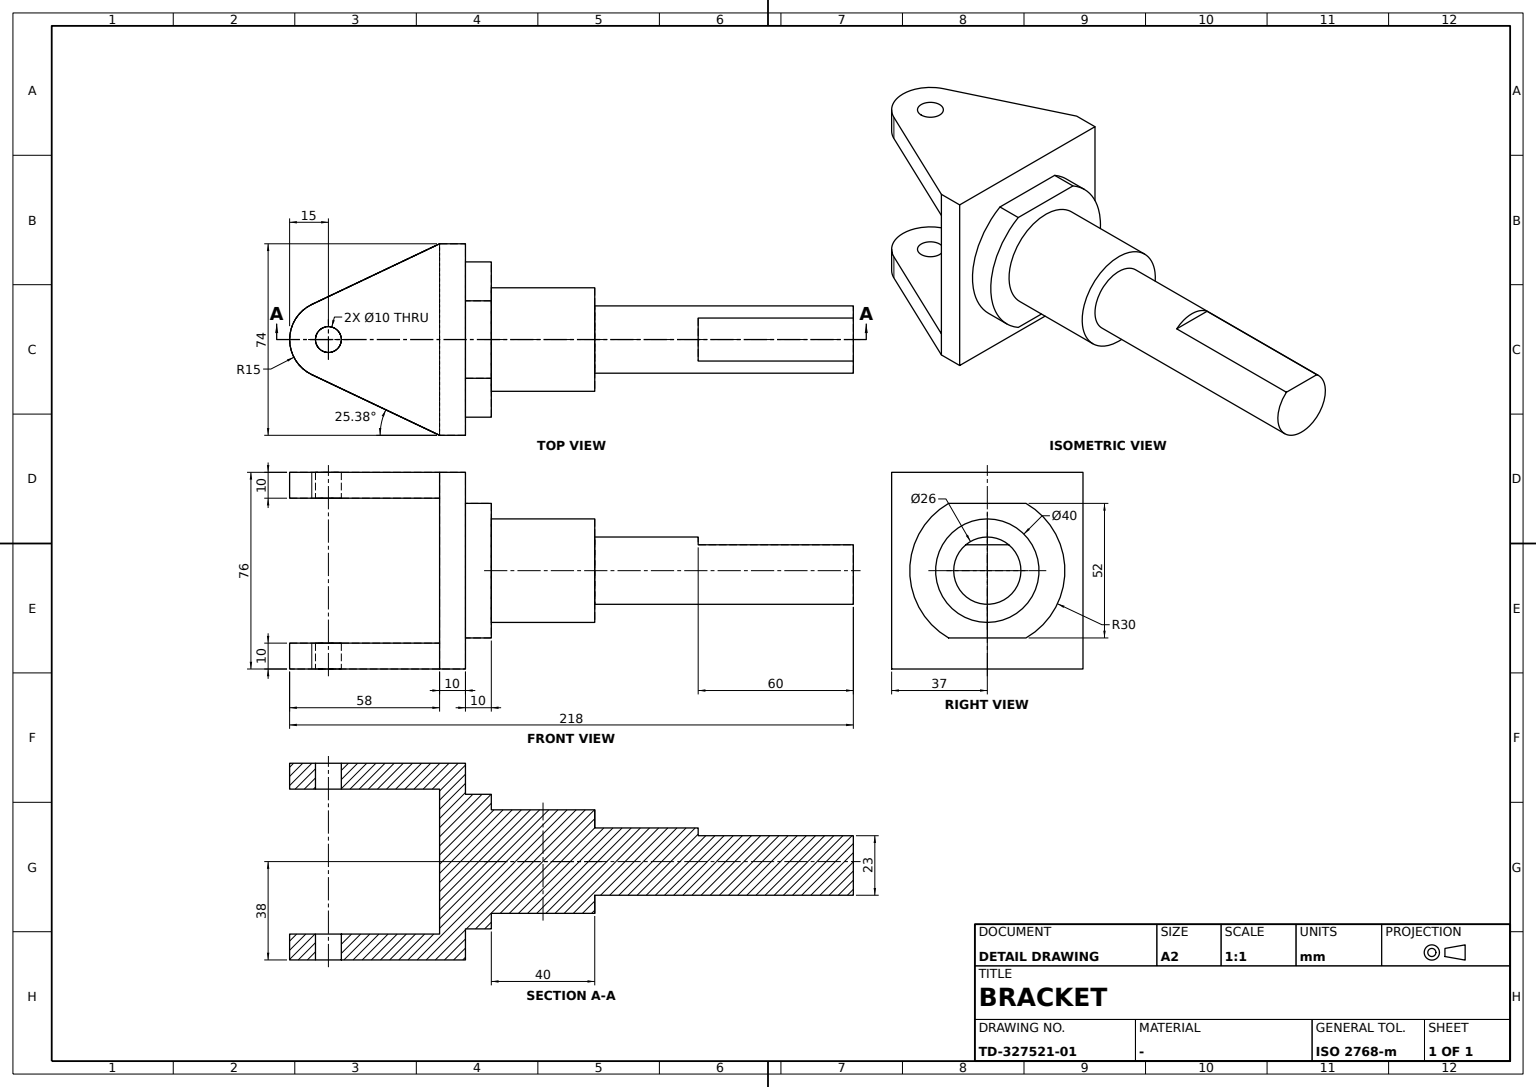
ISO-10303-21;
HEADER;
FILE_DESCRIPTION((''),'2;1');
FILE_NAME('','',(''),(''),'','','');
FILE_SCHEMA(('AUTOMOTIVE_DESIGN'));
ENDSEC;
DATA;
#1=APPLICATION_CONTEXT('');
#2=PRODUCT_CONTEXT('',#1,'mechanical');
#3=PRODUCT('','','',(#2));
#4=PRODUCT_DEFINITION_FORMATION('','',#3);
#5=PRODUCT_DEFINITION_CONTEXT('',#1,'design');
#6=PRODUCT_DEFINITION('','',#4,#5);
#7=PRODUCT_DEFINITION_SHAPE('','',#6);
#8=(LENGTH_UNIT()NAMED_UNIT(*)SI_UNIT(.MILLI.,.METRE.));
#9=(NAMED_UNIT(*)PLANE_ANGLE_UNIT()SI_UNIT($,.RADIAN.));
#10=(NAMED_UNIT(*)SI_UNIT($,.STERADIAN.)SOLID_ANGLE_UNIT());
#11=UNCERTAINTY_MEASURE_WITH_UNIT(LENGTH_MEASURE(0.005),#8,'distance_accuracy_value','');
#12=(GEOMETRIC_REPRESENTATION_CONTEXT(3)GLOBAL_UNCERTAINTY_ASSIGNED_CONTEXT((#11))GLOBAL_UNIT_ASSIGNED_CONTEXT((#8,#9,#10))REPRESENTATION_CONTEXT('',''));
#13=CARTESIAN_POINT('',(13.552475,-149.428874,-38.));
#14=VERTEX_POINT('',#13);
#15=CARTESIAN_POINT('',(37.,-100.,-38.));
#16=VERTEX_POINT('',#15);
#17=DIRECTION('',(0.428591593,0.903498338,0.));
#18=VECTOR('',#17,1000.);
#19=LINE('',#13,#18);
#20=EDGE_CURVE('',#14,#16,#19,.T.);
#21=ORIENTED_EDGE('',*,*,#20,.F.);
#22=CARTESIAN_POINT('',(-13.552475,-149.428874,-38.));
#23=VERTEX_POINT('',#22);
#24=CARTESIAN_POINT('',(0.,-143.,-38.));
#25=DIRECTION('',(0.,0.,1.));
#26=DIRECTION('',(1.,0.,0.));
#27=AXIS2_PLACEMENT_3D('',#24,#25,#26);
#28=CIRCLE('',#27,15.);
#29=EDGE_CURVE('',#14,#23,#28,.F.);
#30=ORIENTED_EDGE('',*,*,#29,.T.);
#31=CARTESIAN_POINT('',(-37.,-100.,-38.));
#32=VERTEX_POINT('',#31);
#33=DIRECTION('',(-0.428591593,0.903498338,0.));
#34=VECTOR('',#33,1000.);
#35=LINE('',#22,#34);
#36=EDGE_CURVE('',#23,#32,#35,.T.);
#37=ORIENTED_EDGE('',*,*,#36,.T.);
#38=CARTESIAN_POINT('',(-37.,-90.,-38.));
#39=VERTEX_POINT('',#38);
#40=DIRECTION('',(0.,-1.,0.));
#41=VECTOR('',#40,1000.);
#42=LINE('',#38,#41);
#43=EDGE_CURVE('',#39,#32,#42,.T.);
#44=ORIENTED_EDGE('',*,*,#43,.F.);
#45=CARTESIAN_POINT('',(37.,-90.,-38.));
#46=VERTEX_POINT('',#45);
#47=CARTESIAN_POINT('',(0.,-90.,-38.));
#48=DIRECTION('',(-1.,0.,0.));
#49=VECTOR('',#48,1000.);
#50=LINE('',#47,#49);
#51=EDGE_CURVE('',#46,#39,#50,.T.);
#52=ORIENTED_EDGE('',*,*,#51,.F.);
#53=LINE('',#45,#41);
#54=EDGE_CURVE('',#46,#16,#53,.T.);
#55=ORIENTED_EDGE('',*,*,#54,.T.);
#56=EDGE_LOOP('',(#21,#30,#37,#44,#52,#55));
#57=FACE_BOUND('',#56,.T.);
#58=CARTESIAN_POINT('',(5.,-143.,-38.));
#59=VERTEX_POINT('',#58);
#60=CIRCLE('',#27,5.);
#61=EDGE_CURVE('',#59,#59,#60,.F.);
#62=ORIENTED_EDGE('',*,*,#61,.F.);
#63=EDGE_LOOP('',(#62));
#64=FACE_BOUND('',#63,.T.);
#65=AXIS2_PLACEMENT_3D('',#45,#25,#48);
#66=PLANE('',#65);
#67=ADVANCED_FACE('',(#57,#64),#66,.F.);
#68=CARTESIAN_POINT('',(8.306624,0.,10.));
#69=VERTEX_POINT('',#68);
#70=CARTESIAN_POINT('',(-8.306624,0.,10.));
#71=VERTEX_POINT('',#70);
#72=CARTESIAN_POINT('',(0.,0.,0.));
#73=DIRECTION('',(0.,1.,0.));
#74=AXIS2_PLACEMENT_3D('',#72,#73,#25);
#75=CIRCLE('',#74,13.);
#76=EDGE_CURVE('',#69,#71,#75,.F.);
#77=ORIENTED_EDGE('',*,*,#76,.F.);
#78=CARTESIAN_POINT('',(0.,0.,10.));
#79=VECTOR('',#26,1000.);
#80=LINE('',#78,#79);
#81=EDGE_CURVE('',#71,#69,#80,.T.);
#82=ORIENTED_EDGE('',*,*,#81,.F.);
#83=EDGE_LOOP('',(#77,#82));
#84=FACE_BOUND('',#83,.T.);
#85=AXIS2_PLACEMENT_3D('',#72,#73,#48);
#86=PLANE('',#85);
#87=ADVANCED_FACE('',(#84),#86,.T.);
#88=CARTESIAN_POINT('',(8.306624,60.,10.));
#89=VERTEX_POINT('',#88);
#90=CARTESIAN_POINT('',(-8.306624,60.,10.));
#91=VERTEX_POINT('',#90);
#92=CARTESIAN_POINT('',(0.,60.,0.));
#93=AXIS2_PLACEMENT_3D('',#92,#73,#25);
#94=CIRCLE('',#93,13.);
#95=EDGE_CURVE('',#89,#91,#94,.T.);
#96=ORIENTED_EDGE('',*,*,#95,.T.);
#97=CARTESIAN_POINT('',(0.,60.,10.));
#98=LINE('',#97,#79);
#99=EDGE_CURVE('',#91,#89,#98,.T.);
#100=ORIENTED_EDGE('',*,*,#99,.T.);
#101=EDGE_LOOP('',(#96,#100));
#102=FACE_BOUND('',#101,.T.);
#103=AXIS2_PLACEMENT_3D('',#92,#73,#48);
#104=PLANE('',#103);
#105=ADVANCED_FACE('',(#102),#104,.T.);
#106=CARTESIAN_POINT('',(-37.,-100.,-28.));
#107=VERTEX_POINT('',#106);
#108=CARTESIAN_POINT('',(-37.,-100.,28.));
#109=VERTEX_POINT('',#108);
#110=CARTESIAN_POINT('',(-37.,-100.,0.));
#111=VECTOR('',#25,1000.);
#112=LINE('',#110,#111);
#113=EDGE_CURVE('',#107,#109,#112,.T.);
#114=ORIENTED_EDGE('',*,*,#113,.T.);
#115=CARTESIAN_POINT('',(-37.,-100.,38.));
#116=VERTEX_POINT('',#115);
#117=DIRECTION('',(0.,0.,-1.));
#118=VECTOR('',#117,1000.);
#119=LINE('',#31,#118);
#120=EDGE_CURVE('',#116,#109,#119,.T.);
#121=ORIENTED_EDGE('',*,*,#120,.F.);
#122=CARTESIAN_POINT('',(-37.,-90.,38.));
#123=VERTEX_POINT('',#122);
#124=LINE('',#122,#41);
#125=EDGE_CURVE('',#123,#116,#124,.T.);
#126=ORIENTED_EDGE('',*,*,#125,.F.);
#127=CARTESIAN_POINT('',(-37.,-90.,0.));
#128=LINE('',#127,#111);
#129=EDGE_CURVE('',#39,#123,#128,.T.);
#130=ORIENTED_EDGE('',*,*,#129,.F.);
#131=ORIENTED_EDGE('',*,*,#43,.T.);
#132=LINE('',#115,#111);
#133=EDGE_CURVE('',#32,#107,#132,.T.);
#134=ORIENTED_EDGE('',*,*,#133,.T.);
#135=EDGE_LOOP('',(#114,#121,#126,#130,#131,#134));
#136=FACE_BOUND('',#135,.T.);
#137=AXIS2_PLACEMENT_3D('',#38,#26,#25);
#138=PLANE('',#137);
#139=ADVANCED_FACE('',(#136),#138,.F.);
#140=CARTESIAN_POINT('',(-13.552475,-149.428874,-28.));
#141=VERTEX_POINT('',#140);
#142=CARTESIAN_POINT('',(-13.552475,-149.428874,-33.));
#143=LINE('',#142,#118);
#144=EDGE_CURVE('',#23,#141,#143,.F.);
#145=ORIENTED_EDGE('',*,*,#144,.T.);
#146=CARTESIAN_POINT('',(-68.926621,-32.696652,-28.));
#147=LINE('',#146,#34);
#148=EDGE_CURVE('',#141,#107,#147,.T.);
#149=ORIENTED_EDGE('',*,*,#148,.T.);
#150=ORIENTED_EDGE('',*,*,#133,.F.);
#151=ORIENTED_EDGE('',*,*,#36,.F.);
#152=EDGE_LOOP('',(#145,#149,#150,#151));
#153=FACE_BOUND('',#152,.T.);
#154=CARTESIAN_POINT('',(-13.552475,-149.428874,38.));
#155=DIRECTION('',(-0.903498338,-0.428591593,0.));
#156=AXIS2_PLACEMENT_3D('',#154,#155,#33);
#157=PLANE('',#156);
#158=ADVANCED_FACE('',(#153),#157,.T.);
#159=ORIENTED_EDGE('',*,*,#29,.F.);
#160=CARTESIAN_POINT('',(13.552475,-149.428874,-28.));
#161=VERTEX_POINT('',#160);
#162=CARTESIAN_POINT('',(13.552475,-149.428874,-33.));
#163=LINE('',#162,#118);
#164=EDGE_CURVE('',#14,#161,#163,.F.);
#165=ORIENTED_EDGE('',*,*,#164,.T.);
#166=CARTESIAN_POINT('',(0.,-143.,-28.));
#167=AXIS2_PLACEMENT_3D('',#166,#117,#48);
#168=CIRCLE('',#167,15.);
#169=EDGE_CURVE('',#161,#141,#168,.T.);
#170=ORIENTED_EDGE('',*,*,#169,.T.);
#171=ORIENTED_EDGE('',*,*,#144,.F.);
#172=EDGE_LOOP('',(#159,#165,#170,#171));
#173=FACE_BOUND('',#172,.T.);
#174=CARTESIAN_POINT('',(0.,-143.,-33.));
#175=AXIS2_PLACEMENT_3D('',#174,#117,#26);
#176=CYLINDRICAL_SURFACE('',#175,15.);
#177=ADVANCED_FACE('',(#173),#176,.T.);
#178=CARTESIAN_POINT('',(14.96663,-80.,26.));
#179=VERTEX_POINT('',#178);
#180=CARTESIAN_POINT('',(-14.96663,-80.,26.));
#181=VERTEX_POINT('',#180);
#182=CARTESIAN_POINT('',(0.,-80.,26.));
#183=LINE('',#182,#49);
#184=EDGE_CURVE('',#179,#181,#183,.T.);
#185=ORIENTED_EDGE('',*,*,#184,.T.);
#186=CARTESIAN_POINT('',(-14.96663,-90.,26.));
#187=VERTEX_POINT('',#186);
#188=LINE('',#180,#41);
#189=EDGE_CURVE('',#181,#187,#188,.T.);
#190=ORIENTED_EDGE('',*,*,#189,.T.);
#191=CARTESIAN_POINT('',(14.96663,-90.,26.));
#192=VERTEX_POINT('',#191);
#193=CARTESIAN_POINT('',(0.,-90.,26.));
#194=LINE('',#193,#49);
#195=EDGE_CURVE('',#192,#187,#194,.T.);
#196=ORIENTED_EDGE('',*,*,#195,.F.);
#197=LINE('',#178,#41);
#198=EDGE_CURVE('',#179,#192,#197,.T.);
#199=ORIENTED_EDGE('',*,*,#198,.F.);
#200=EDGE_LOOP('',(#185,#190,#196,#199));
#201=FACE_BOUND('',#200,.T.);
#202=AXIS2_PLACEMENT_3D('',#178,#25,#48);
#203=PLANE('',#202);
#204=ADVANCED_FACE('',(#201),#203,.T.);
#205=CARTESIAN_POINT('',(-13.552475,-149.428874,28.));
#206=VERTEX_POINT('',#205);
#207=CARTESIAN_POINT('',(13.552476,-149.428871,28.));
#208=VERTEX_POINT('',#207);
#209=CARTESIAN_POINT('',(0.,-143.,28.));
#210=AXIS2_PLACEMENT_3D('',#209,#25,#26);
#211=CIRCLE('',#210,15.);
#212=EDGE_CURVE('',#206,#208,#211,.T.);
#213=ORIENTED_EDGE('',*,*,#212,.T.);
#214=CARTESIAN_POINT('',(13.552475,-149.428874,38.));
#215=VERTEX_POINT('',#214);
#216=EDGE_CURVE('',#215,#208,#163,.T.);
#217=ORIENTED_EDGE('',*,*,#216,.F.);
#218=CARTESIAN_POINT('',(-13.552476,-149.428871,38.));
#219=VERTEX_POINT('',#218);
#220=CARTESIAN_POINT('',(0.,-143.,38.));
#221=AXIS2_PLACEMENT_3D('',#220,#117,#48);
#222=CIRCLE('',#221,15.);
#223=EDGE_CURVE('',#219,#215,#222,.F.);
#224=ORIENTED_EDGE('',*,*,#223,.F.);
#225=EDGE_CURVE('',#219,#206,#143,.T.);
#226=ORIENTED_EDGE('',*,*,#225,.T.);
#227=EDGE_LOOP('',(#213,#217,#224,#226));
#228=FACE_BOUND('',#227,.T.);
#229=ADVANCED_FACE('',(#228),#176,.T.);
#230=CARTESIAN_POINT('',(0.,-40.,-20.));
#231=VERTEX_POINT('',#230);
#232=CARTESIAN_POINT('',(0.,-40.,0.));
#233=AXIS2_PLACEMENT_3D('',#232,#40,#117);
#234=CIRCLE('',#233,20.);
#235=EDGE_CURVE('',#231,#231,#234,.T.);
#236=ORIENTED_EDGE('',*,*,#235,.F.);
#237=EDGE_LOOP('',(#236));
#238=FACE_BOUND('',#237,.T.);
#239=CARTESIAN_POINT('',(0.,-40.,-13.));
#240=VERTEX_POINT('',#239);
#241=CIRCLE('',#233,13.);
#242=EDGE_CURVE('',#240,#240,#241,.T.);
#243=ORIENTED_EDGE('',*,*,#242,.T.);
#244=EDGE_LOOP('',(#243));
#245=FACE_BOUND('',#244,.T.);
#246=AXIS2_PLACEMENT_3D('',#232,#40,#26);
#247=PLANE('',#246);
#248=ADVANCED_FACE('',(#238,#245),#247,.F.);
#249=CARTESIAN_POINT('',(0.,-80.,-20.));
#250=VERTEX_POINT('',#249);
#251=CARTESIAN_POINT('',(0.,-80.,0.));
#252=AXIS2_PLACEMENT_3D('',#251,#40,#117);
#253=CIRCLE('',#252,20.);
#254=EDGE_CURVE('',#250,#250,#253,.T.);
#255=ORIENTED_EDGE('',*,*,#254,.T.);
#256=EDGE_LOOP('',(#255));
#257=FACE_BOUND('',#256,.T.);
#258=CARTESIAN_POINT('',(14.96663,-80.,-26.));
#259=VERTEX_POINT('',#258);
#260=CIRCLE('',#252,30.);
#261=EDGE_CURVE('',#259,#179,#260,.T.);
#262=ORIENTED_EDGE('',*,*,#261,.F.);
#263=CARTESIAN_POINT('',(-14.96663,-80.,-26.));
#264=VERTEX_POINT('',#263);
#265=CARTESIAN_POINT('',(0.,-80.,-26.));
#266=LINE('',#265,#49);
#267=EDGE_CURVE('',#259,#264,#266,.T.);
#268=ORIENTED_EDGE('',*,*,#267,.T.);
#269=EDGE_CURVE('',#181,#264,#260,.T.);
#270=ORIENTED_EDGE('',*,*,#269,.F.);
#271=ORIENTED_EDGE('',*,*,#184,.F.);
#272=EDGE_LOOP('',(#262,#268,#270,#271));
#273=FACE_BOUND('',#272,.T.);
#274=AXIS2_PLACEMENT_3D('',#251,#40,#26);
#275=PLANE('',#274);
#276=ADVANCED_FACE('',(#257,#273),#275,.F.);
#277=CARTESIAN_POINT('',(14.96663,-90.,-26.));
#278=VERTEX_POINT('',#277);
#279=CARTESIAN_POINT('',(0.,-90.,0.));
#280=AXIS2_PLACEMENT_3D('',#279,#40,#117);
#281=CIRCLE('',#280,30.);
#282=EDGE_CURVE('',#278,#192,#281,.T.);
#283=ORIENTED_EDGE('',*,*,#282,.T.);
#284=ORIENTED_EDGE('',*,*,#195,.T.);
#285=CARTESIAN_POINT('',(-14.96663,-90.,-26.));
#286=VERTEX_POINT('',#285);
#287=EDGE_CURVE('',#187,#286,#281,.T.);
#288=ORIENTED_EDGE('',*,*,#287,.T.);
#289=CARTESIAN_POINT('',(0.,-90.,-26.));
#290=LINE('',#289,#49);
#291=EDGE_CURVE('',#278,#286,#290,.T.);
#292=ORIENTED_EDGE('',*,*,#291,.F.);
#293=EDGE_LOOP('',(#283,#284,#288,#292));
#294=FACE_BOUND('',#293,.T.);
#295=ORIENTED_EDGE('',*,*,#129,.T.);
#296=CARTESIAN_POINT('',(37.,-90.,38.));
#297=VERTEX_POINT('',#296);
#298=CARTESIAN_POINT('',(0.,-90.,38.));
#299=LINE('',#298,#79);
#300=EDGE_CURVE('',#123,#297,#299,.T.);
#301=ORIENTED_EDGE('',*,*,#300,.T.);
#302=CARTESIAN_POINT('',(37.,-90.,0.));
#303=LINE('',#302,#118);
#304=EDGE_CURVE('',#297,#46,#303,.T.);
#305=ORIENTED_EDGE('',*,*,#304,.T.);
#306=ORIENTED_EDGE('',*,*,#51,.T.);
#307=EDGE_LOOP('',(#295,#301,#305,#306));
#308=FACE_BOUND('',#307,.T.);
#309=AXIS2_PLACEMENT_3D('',#279,#40,#26);
#310=PLANE('',#309);
#311=ADVANCED_FACE('',(#294,#308),#310,.F.);
#312=CARTESIAN_POINT('',(37.,-100.,28.));
#313=VERTEX_POINT('',#312);
#314=CARTESIAN_POINT('',(13.552475,-149.428874,28.));
#315=LINE('',#314,#18);
#316=EDGE_CURVE('',#208,#313,#315,.T.);
#317=ORIENTED_EDGE('',*,*,#316,.F.);
#318=ORIENTED_EDGE('',*,*,#212,.F.);
#319=LINE('',#205,#34);
#320=EDGE_CURVE('',#206,#109,#319,.T.);
#321=ORIENTED_EDGE('',*,*,#320,.T.);
#322=CARTESIAN_POINT('',(0.,-100.,28.));
#323=LINE('',#322,#79);
#324=EDGE_CURVE('',#109,#313,#323,.T.);
#325=ORIENTED_EDGE('',*,*,#324,.T.);
#326=EDGE_LOOP('',(#317,#318,#321,#325));
#327=FACE_BOUND('',#326,.T.);
#328=CARTESIAN_POINT('',(5.,-143.,28.));
#329=VERTEX_POINT('',#328);
#330=CIRCLE('',#210,5.);
#331=EDGE_CURVE('',#329,#329,#330,.T.);
#332=ORIENTED_EDGE('',*,*,#331,.T.);
#333=EDGE_LOOP('',(#332));
#334=FACE_BOUND('',#333,.T.);
#335=CARTESIAN_POINT('',(0.,0.,28.));
#336=AXIS2_PLACEMENT_3D('',#335,#25,#26);
#337=PLANE('',#336);
#338=ADVANCED_FACE('',(#327,#334),#337,.F.);
#339=CARTESIAN_POINT('',(-5.,-143.,-28.));
#340=VERTEX_POINT('',#339);
#341=CIRCLE('',#167,5.);
#342=EDGE_CURVE('',#340,#340,#341,.T.);
#343=ORIENTED_EDGE('',*,*,#342,.F.);
#344=EDGE_LOOP('',(#343));
#345=FACE_BOUND('',#344,.T.);
#346=ORIENTED_EDGE('',*,*,#61,.T.);
#347=EDGE_LOOP('',(#346));
#348=FACE_BOUND('',#347,.T.);
#349=CYLINDRICAL_SURFACE('',#175,5.);
#350=ADVANCED_FACE('',(#345,#348),#349,.F.);
#351=ORIENTED_EDGE('',*,*,#254,.F.);
#352=EDGE_LOOP('',(#351));
#353=FACE_BOUND('',#352,.T.);
#354=ORIENTED_EDGE('',*,*,#235,.T.);
#355=EDGE_LOOP('',(#354));
#356=FACE_BOUND('',#355,.T.);
#357=CARTESIAN_POINT('',(0.,-60.,0.));
#358=AXIS2_PLACEMENT_3D('',#357,#40,#26);
#359=CYLINDRICAL_SURFACE('',#358,20.);
#360=ADVANCED_FACE('',(#353,#356),#359,.T.);
#361=ORIENTED_EDGE('',*,*,#287,.F.);
#362=ORIENTED_EDGE('',*,*,#189,.F.);
#363=ORIENTED_EDGE('',*,*,#269,.T.);
#364=LINE('',#263,#41);
#365=EDGE_CURVE('',#264,#286,#364,.T.);
#366=ORIENTED_EDGE('',*,*,#365,.T.);
#367=EDGE_LOOP('',(#361,#362,#363,#366));
#368=FACE_BOUND('',#367,.T.);
#369=CARTESIAN_POINT('',(0.,-85.,0.));
#370=AXIS2_PLACEMENT_3D('',#369,#40,#26);
#371=CYLINDRICAL_SURFACE('',#370,30.);
#372=ADVANCED_FACE('',(#368),#371,.T.);
#373=LINE('',#68,#41);
#374=EDGE_CURVE('',#89,#69,#373,.T.);
#375=ORIENTED_EDGE('',*,*,#374,.T.);
#376=ORIENTED_EDGE('',*,*,#76,.T.);
#377=LINE('',#70,#41);
#378=EDGE_CURVE('',#71,#91,#377,.F.);
#379=ORIENTED_EDGE('',*,*,#378,.T.);
#380=ORIENTED_EDGE('',*,*,#95,.F.);
#381=EDGE_LOOP('',(#375,#376,#379,#380));
#382=FACE_BOUND('',#381,.T.);
#383=ORIENTED_EDGE('',*,*,#242,.F.);
#384=EDGE_LOOP('',(#383));
#385=FACE_BOUND('',#384,.T.);
#386=CARTESIAN_POINT('',(0.,-20.,0.));
#387=AXIS2_PLACEMENT_3D('',#386,#40,#26);
#388=CYLINDRICAL_SURFACE('',#387,13.);
#389=ADVANCED_FACE('',(#382,#385),#388,.T.);
#390=ORIENTED_EDGE('',*,*,#99,.F.);
#391=ORIENTED_EDGE('',*,*,#378,.F.);
#392=ORIENTED_EDGE('',*,*,#81,.T.);
#393=ORIENTED_EDGE('',*,*,#374,.F.);
#394=EDGE_LOOP('',(#390,#391,#392,#393));
#395=FACE_BOUND('',#394,.T.);
#396=AXIS2_PLACEMENT_3D('',#70,#25,#26);
#397=PLANE('',#396);
#398=ADVANCED_FACE('',(#395),#397,.T.);
#399=ORIENTED_EDGE('',*,*,#324,.F.);
#400=ORIENTED_EDGE('',*,*,#113,.F.);
#401=CARTESIAN_POINT('',(37.,-100.,-28.));
#402=VERTEX_POINT('',#401);
#403=CARTESIAN_POINT('',(0.,-100.,-28.));
#404=LINE('',#403,#79);
#405=EDGE_CURVE('',#107,#402,#404,.T.);
#406=ORIENTED_EDGE('',*,*,#405,.T.);
#407=CARTESIAN_POINT('',(37.,-100.,0.));
#408=LINE('',#407,#118);
#409=EDGE_CURVE('',#313,#402,#408,.T.);
#410=ORIENTED_EDGE('',*,*,#409,.F.);
#411=EDGE_LOOP('',(#399,#400,#406,#410));
#412=FACE_BOUND('',#411,.T.);
#413=CARTESIAN_POINT('',(0.,-100.,0.));
#414=AXIS2_PLACEMENT_3D('',#413,#40,#26);
#415=PLANE('',#414);
#416=ADVANCED_FACE('',(#412),#415,.T.);
#417=ORIENTED_EDGE('',*,*,#291,.T.);
#418=ORIENTED_EDGE('',*,*,#365,.F.);
#419=ORIENTED_EDGE('',*,*,#267,.F.);
#420=LINE('',#258,#41);
#421=EDGE_CURVE('',#259,#278,#420,.T.);
#422=ORIENTED_EDGE('',*,*,#421,.T.);
#423=EDGE_LOOP('',(#417,#418,#419,#422));
#424=FACE_BOUND('',#423,.T.);
#425=AXIS2_PLACEMENT_3D('',#258,#25,#48);
#426=PLANE('',#425);
#427=ADVANCED_FACE('',(#424),#426,.F.);
#428=CARTESIAN_POINT('',(37.,-100.,38.));
#429=LINE('',#428,#111);
#430=EDGE_CURVE('',#16,#402,#429,.T.);
#431=ORIENTED_EDGE('',*,*,#430,.F.);
#432=ORIENTED_EDGE('',*,*,#54,.F.);
#433=ORIENTED_EDGE('',*,*,#304,.F.);
#434=VERTEX_POINT('',#428);
#435=LINE('',#296,#41);
#436=EDGE_CURVE('',#297,#434,#435,.T.);
#437=ORIENTED_EDGE('',*,*,#436,.T.);
#438=LINE('',#428,#118);
#439=EDGE_CURVE('',#434,#313,#438,.T.);
#440=ORIENTED_EDGE('',*,*,#439,.T.);
#441=ORIENTED_EDGE('',*,*,#409,.T.);
#442=EDGE_LOOP('',(#431,#432,#433,#437,#440,#441));
#443=FACE_BOUND('',#442,.T.);
#444=AXIS2_PLACEMENT_3D('',#296,#48,#117);
#445=PLANE('',#444);
#446=ADVANCED_FACE('',(#443),#445,.F.);
#447=CARTESIAN_POINT('',(-5.,-143.,38.));
#448=VERTEX_POINT('',#447);
#449=CIRCLE('',#221,5.);
#450=EDGE_CURVE('',#448,#448,#449,.F.);
#451=ORIENTED_EDGE('',*,*,#450,.F.);
#452=EDGE_LOOP('',(#451));
#453=FACE_BOUND('',#452,.T.);
#454=ORIENTED_EDGE('',*,*,#125,.T.);
#455=CARTESIAN_POINT('',(-40.872318,-91.836908,38.));
#456=LINE('',#455,#34);
#457=EDGE_CURVE('',#219,#116,#456,.T.);
#458=ORIENTED_EDGE('',*,*,#457,.F.);
#459=ORIENTED_EDGE('',*,*,#223,.T.);
#460=CARTESIAN_POINT('',(27.279202,-120.49206,38.));
#461=LINE('',#460,#18);
#462=EDGE_CURVE('',#215,#434,#461,.T.);
#463=ORIENTED_EDGE('',*,*,#462,.T.);
#464=ORIENTED_EDGE('',*,*,#436,.F.);
#465=ORIENTED_EDGE('',*,*,#300,.F.);
#466=EDGE_LOOP('',(#454,#458,#459,#463,#464,#465));
#467=FACE_BOUND('',#466,.T.);
#468=AXIS2_PLACEMENT_3D('',#122,#117,#26);
#469=PLANE('',#468);
#470=ADVANCED_FACE('',(#453,#467),#469,.F.);
#471=ORIENTED_EDGE('',*,*,#439,.F.);
#472=ORIENTED_EDGE('',*,*,#462,.F.);
#473=ORIENTED_EDGE('',*,*,#216,.T.);
#474=ORIENTED_EDGE('',*,*,#316,.T.);
#475=EDGE_LOOP('',(#471,#472,#473,#474));
#476=FACE_BOUND('',#475,.T.);
#477=DIRECTION('',(-0.903498338,0.428591593,0.));
#478=AXIS2_PLACEMENT_3D('',#214,#477,#17);
#479=PLANE('',#478);
#480=ADVANCED_FACE('',(#476),#479,.F.);
#481=CARTESIAN_POINT('',(68.926621,-32.696652,-28.));
#482=LINE('',#481,#18);
#483=EDGE_CURVE('',#161,#402,#482,.T.);
#484=ORIENTED_EDGE('',*,*,#483,.F.);
#485=ORIENTED_EDGE('',*,*,#164,.F.);
#486=ORIENTED_EDGE('',*,*,#20,.T.);
#487=ORIENTED_EDGE('',*,*,#430,.T.);
#488=EDGE_LOOP('',(#484,#485,#486,#487));
#489=FACE_BOUND('',#488,.T.);
#490=ADVANCED_FACE('',(#489),#479,.F.);
#491=ORIENTED_EDGE('',*,*,#320,.F.);
#492=ORIENTED_EDGE('',*,*,#225,.F.);
#493=ORIENTED_EDGE('',*,*,#457,.T.);
#494=ORIENTED_EDGE('',*,*,#120,.T.);
#495=EDGE_LOOP('',(#491,#492,#493,#494));
#496=FACE_BOUND('',#495,.T.);
#497=ADVANCED_FACE('',(#496),#157,.T.);
#498=ORIENTED_EDGE('',*,*,#450,.T.);
#499=EDGE_LOOP('',(#498));
#500=FACE_BOUND('',#499,.T.);
#501=ORIENTED_EDGE('',*,*,#331,.F.);
#502=EDGE_LOOP('',(#501));
#503=FACE_BOUND('',#502,.T.);
#504=ADVANCED_FACE('',(#500,#503),#349,.F.);
#505=ORIENTED_EDGE('',*,*,#342,.T.);
#506=EDGE_LOOP('',(#505));
#507=FACE_BOUND('',#506,.T.);
#508=ORIENTED_EDGE('',*,*,#483,.T.);
#509=ORIENTED_EDGE('',*,*,#405,.F.);
#510=ORIENTED_EDGE('',*,*,#148,.F.);
#511=ORIENTED_EDGE('',*,*,#169,.F.);
#512=EDGE_LOOP('',(#508,#509,#510,#511));
#513=FACE_BOUND('',#512,.T.);
#514=CARTESIAN_POINT('',(0.,0.,-28.));
#515=AXIS2_PLACEMENT_3D('',#514,#117,#26);
#516=PLANE('',#515);
#517=ADVANCED_FACE('',(#507,#513),#516,.F.);
#518=ORIENTED_EDGE('',*,*,#282,.F.);
#519=ORIENTED_EDGE('',*,*,#421,.F.);
#520=ORIENTED_EDGE('',*,*,#261,.T.);
#521=ORIENTED_EDGE('',*,*,#198,.T.);
#522=EDGE_LOOP('',(#518,#519,#520,#521));
#523=FACE_BOUND('',#522,.T.);
#524=ADVANCED_FACE('',(#523),#371,.T.);
#525=CLOSED_SHELL('',(#67,#87,#105,#139,#158,#177,#204,#229,#248,#276,#311,#338,#350,#360,#372,#389,#398,#416,#427,#446,#470,#480,#490,#497,#504,#517,#524));
#526=MANIFOLD_SOLID_BREP('',#525);
#527=ADVANCED_BREP_SHAPE_REPRESENTATION('',(#526),#12);
#528=SHAPE_DEFINITION_REPRESENTATION(#7,#527);
ENDSEC;
END-ISO-10303-21;
